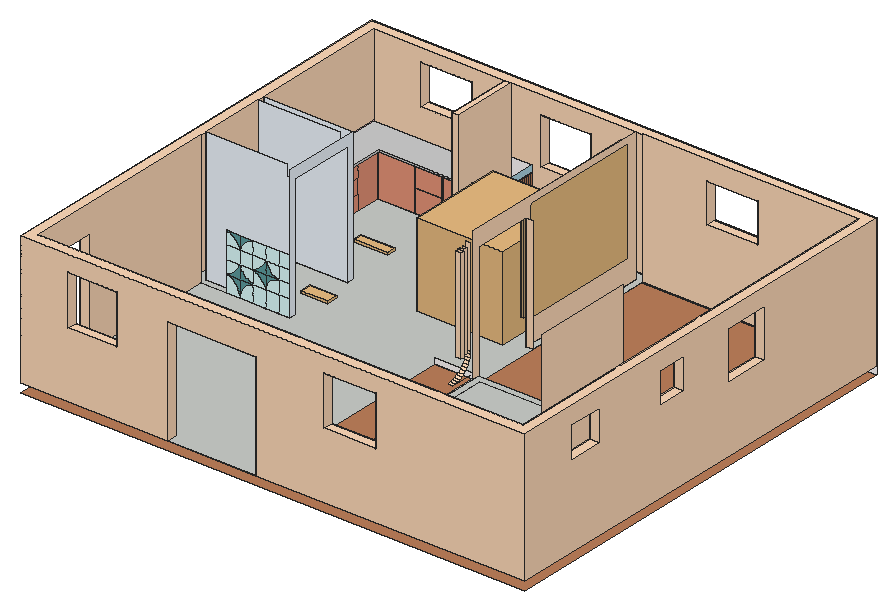
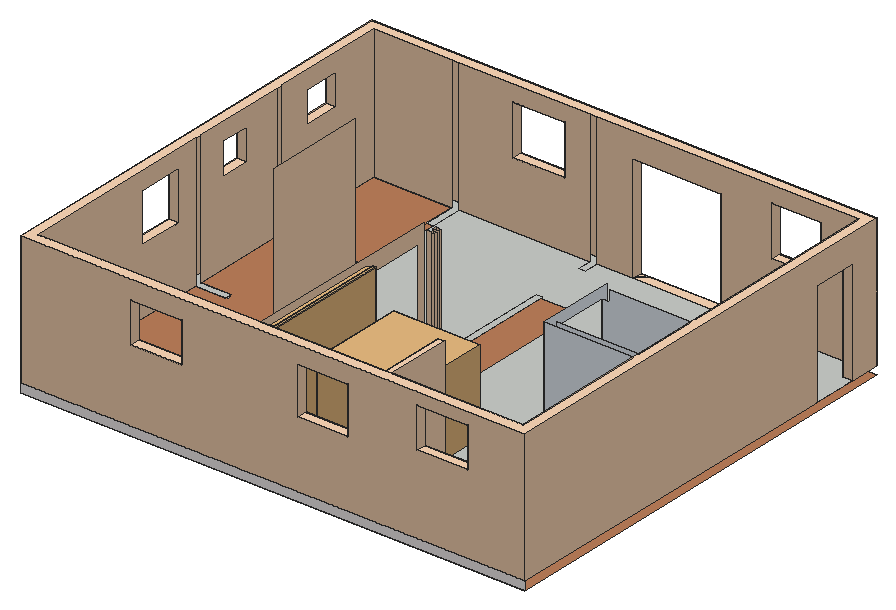
# SketchUp Ruby script. Lengths in inches.
U = 1.inch
M = Sketchup.active_model
def pt(a) = Geom::Point3d.new(a.map { |v| v * U })
def face(e, loops, mat)
  f = e.add_face(loops[0].map { |a| pt(a) })
  loops[1..].each { |l| e.add_face(l.map { |a| pt(a) }).erase! }
  f.material = f.back_material = mat if mat
  f
end
# faces: each face lists its corners as indices into pts; further lists are holes
def faces(e, pts, list, mat = nil) = list.each { |f| face(e, (f[0].is_a?(Array) ? f : [f]).map { |l| l.map { |i| pts[i] } }, mat) }
# xy, xz, yz: faces in a plane at the given z, y or x. An outline is a flat list of corners, or four numbers for a rectangle; further outlines are holes
def ring(l) = l.size == 4 ? [[l[0], l[1]], [l[2], l[1]], [l[2], l[3]], [l[0], l[3]]] : l.each_slice(2).to_a
def flat(e, list, mat, &to3) = list.each { |f| face(e, (f[0].is_a?(Array) ? f : [f]).map { |l| ring(l).map { |u, v| to3.(u, v) } }, mat) }
def xy(e, z, list, mat = nil) = flat(e, list, mat) { |x, y| [x, y, z] }
def xz(e, y, list, mat = nil) = flat(e, list, mat) { |x, z| [x, y, z] }
def yz(e, x, list, mat = nil) = flat(e, list, mat) { |y, z| [x, y, z] }
def lines(e, pts, list) = list.each { |a, b| e.add_line(pt(pts[a]), pt(pts[b])) }
# prism: a flat outline (further loops are holes) pulled along v
def prism(e, loops, v, mat = nil)
  f = face(e, loops, mat); d = Geom::Vector3d.new(v.map { |x| x * U })
  f.pushpull(f.normal.samedirection?(d) ? d.length : -d.length)
end
def box(e, o, s, mat = nil) = prism(e, [[o, [o[0] + s[0], o[1], o[2]], [o[0] + s[0], o[1] + s[1], o[2]], [o[0], o[1] + s[1], o[2]]]], [0, 0, s[2]], mat)
def at(x, y, z, deg = 0) = Geom::Transformation.translation(pt([x, y, z])) * Geom::Transformation.rotation(ORIGIN, Z_AXIS, deg.degrees)
def axes(o, x, y, z) = Geom::Transformation.new([*x, 0, *y, 0, *z, 0, *pt(o).to_a, 1])
def part(name) = M.definitions.add(name)
# library, detail: a bought-in or finely detailed component or shape, given as its bounding box
def library(name, o, s) = part(name).tap { |d| box(d.entities, o, s) }
def detail(e, o, s) = box(e.add_group.entities, o, s)
def put(e, d, t, mat = nil) = e.add_instance(d, t).tap { |i| i.material = mat if mat }
def group(e, t, mat = nil) = e.add_group.tap { |g| g.transformation = t; g.material = mat if mat }.entities
root = M.entities
M.materials.add("3D66_SU_1584934530570_001").color = [198, 166, 120]
M.materials.add("[0006_Pink]").color = [255, 192, 203]
M.materials.add("[0010_Snow]").color = [255, 250, 250]
M.materials.add("[0014_DarkSalmon]").color = [233, 150, 122]
M.materials.add("[0027_PeachPuff]").color = [255, 218, 185]
M.materials.add("[0081_CadetBlue]").color = [95, 158, 160]
M.materials.add("[0090_LightCyan]").color = [224, 255, 255]
M.materials.add("[0093_AliceBlue]").color = [240, 248, 255]
M.materials.add("[0095_LightBlue]").color = [173, 216, 230]
M.materials.add("[Basic Tile]").color = [203, 206, 202]
M.materials.add("[Carrera Marble]").color = [207, 207, 207]
M.materials.add("[Wood Veneer 02]").color = [190, 128, 91]
c1 = library("kitchen",[0.875,0,0],[30.86,8.22,2])
c2 = library("pooja",[0.875,0,0],[24.44,10.22,2])
c3 = library("Dining table and chairs",[0,0,0],[63.25,59.01,43.49])
c4 = library("Dining ar",[0.98,0,0],[40.63,10.22,2])
c5 = part("\#79\#1")
prism(c5.entities,[[[1108.05,3703.68,-100.79],[497.03,3703.68,-100.79],[497.03,5166.16,-100.79],[1108.05,5166.16,-100.79]],[[1097.77,5155.88,-100.79],[507.31,5155.88,-100.79],[507.31,3713.96,-100.79],[1097.77,3713.96,-100.79]]],[0,0,14.57],"3D66_SU_1584934530570_001")
c6 = library("\#81",[507.31,3713.96,-116.94],[590.46,1441.92,47.04])
xy(root,-7.5625,[[109.5625,138.9375,571.5625,540.9375]],"[Wood Veneer 02]")
xy(root,0,[[[109.5625,138.9375,571.5625,540.9375],[490.5625,258.9375,490.5625,347.21,492.04,347.21,492.04,350.1875,490.5625,350.1875,490.5625,351.9375,364.5625,351.9375,364.5625,531.9375,562.5625,531.9375,562.5625,351.9375,534.83,351.9375,534.83,350.1875,533.35,350.1875,533.35,348.7,535.05,348.7,535.05,345.9375,562.5625,345.9375,562.5625,258.9375],[490.5625,147.9375,490.5625,177.19,483.52,177.19,483.52,240.51,490.5625,240.51,490.5625,252.9375,562.5625,252.9375,562.5625,147.9375],[323.75,211.625,358.5625,345.9375],[118.5625,405.9375,139.41,531.9375],[244.5625,486.17,263.2,531.9375]]],"[Basic Tile]")
xy(root,6.75,[[263.2,488.05,263.89,509.17],[263.89,488.05,264.76,489.21],[263.89,490.54,264.76,491.71],[263.89,493.04,264.76,494.2],[263.89,495.53,264.76,496.7],
  [263.89,498.03,264.76,499.19],[263.89,500.52,264.76,501.6875],[263.89,503.02,264.76,504.18],[263.89,505.51,264.76,506.68],[263.89,508.01,264.76,509.17],
  [263.2,509.67,263.89,530],[263.89,510.01,264.76,511.17],[263.89,512.36,264.76,513.53],[263.89,514.71,264.76,515.88],[263.89,517.07,264.76,518.23],
  [263.89,519.42,264.76,520.59],[263.89,521.77,264.76,522.9375],[263.89,524.125,264.76,525.29],[263.89,526.48,264.76,527.65],[263.89,528.83,264.76,530]],"[0010_Snow]")
xy(root,23.08,[[354.3125,330.97,359.375,333.97],[354.3125,336.47,357.4375,339.47]],"[0027_PeachPuff]")
xy(root,44.75,[[118.58,405.9375,118.58,533.96,238.5625,533.96,238.5625,500.54,148.4,500.54,148.4,405.9375]],"[0006_Pink]")
xy(root,46.25,[[118.58,405.9375,148.4,405.9375,148.4,500.54,238.5625,500.54,238.5625,533.96,118.58,533.96]],"[Carrera Marble]")
xy(root,121.1875,[[238.5625,471.5,244.5625,531.9375]],"[0027_PeachPuff]")
xz(root,330.97,[[354.3125,23.08,359.375,110.27]],"[0027_PeachPuff]")
xz(root,333.9375,[[154.5625,0,154.5625,15.41,142.5625,15.41,144.1875,14.8125,145.74,14.05,147.22,13.14,148.59,12.09,149.85,10.9,150.98,9.59,151.97,8.17,152.82,6.66,153.5,5.07,154.03,3.42,154.38,1.72],[154.5625,0,154.6875,1.74,155,3.46,155.49,5.13,156.16,6.74,157,8.27,158,9.7,159.14,11.02,160.42,12.2,161.82,13.25,163.32,14.14,164.91,14.86,166.5625,15.41,154.5625,15.41],[142.5625,15.41,154.5625,15.41,154.5625,27.41,154.01,26.06,153.37,24.75,152.625,23.49,151.8,22.29,150.88,21.15,149.89,20.08,148.82,19.09,147.68,18.17,146.48,17.35,145.22,16.61,143.91,15.96],[154.5625,15.41,166.5625,15.41,165.19,15.93,163.86,16.55,162.59,17.27,161.37,18.09,160.22,19,159.15,19.99,158.15,21.07,157.24,22.22,156.42,23.43,155.7,24.71,155.08,26.04,154.5625,27.41],[178.5625,15.41,178.5625,27.41,166.5625,27.41,167.94,26.91,169.28,26.3,170.5625,25.58,171.79,24.77,172.94,23.86,174.02,22.87,175.02,21.79,175.93,20.63,176.74,19.41,177.45,18.125,178.0625,16.79],
  [178.5625,15.41,178.7,16.96,179.04,18.48,179.57,19.95,180.27,21.34,181.15,22.625,182.18,23.79,183.34,24.82,184.63,25.7,186.02,26.4,187.49,26.93,189.01,27.27,190.5625,27.41,178.5625,27.41],[166.5625,27.41,178.5625,27.41,178.5625,39.41,178.01,38.06,177.37,36.75,176.625,35.49,175.8,34.29,174.88,33.15,173.89,32.08,172.82,31.09,171.68,30.17,170.48,29.35,169.22,28.61,167.91,27.96],[178.5625,27.41,190.5625,27.41,189.12,27.79,187.72,28.3125,186.375,28.96,185.1,29.74,183.9,30.64,182.79,31.64,181.79,32.75,180.9,33.94,180.12,35.22,179.47,36.5625,178.95,37.96,178.5625,39.41],[154.5625,39.41,154.5625,51.41,142.5625,51.41,143.91,50.85,145.22,50.21,146.48,49.46,147.68,48.63,148.8125,47.72,149.88,46.73,150.875,45.66,151.79,44.52,152.62,43.32,153.36,42.06,154.01,40.76],[154.5625,39.41,155.0625,40.79,155.67,42.125,156.39,43.41,157.2,44.63,158.11,45.79,159.1,46.87,160.18,47.86,161.34,48.77,162.5625,49.58,163.85,50.3,165.18,50.91,166.5625,51.41,154.5625,51.41]],"[0081_CadetBlue]")
xz(root,333.9375,[[142.5625,0,154.5625,0,154.38,1.72,154.03,3.42,153.5,5.07,152.82,6.66,151.97,8.17,150.98,9.59,149.85,10.9,148.59,12.09,147.22,13.14,145.74,14.05,144.1875,14.8125,142.5625,15.41],[154.5625,0,166.5625,0,166.5625,15.41,164.91,14.86,163.32,14.14,161.82,13.25,160.42,12.2,159.14,11.02,158,9.7,157,8.27,156.16,6.74,155.49,5.13,155,3.46,154.6875,1.74],[166.5625,0,178.5625,15.41],[178.5625,0,190.5625,15.41],[190.5625,0,200.19,15.41],
  [142.5625,15.41,143.91,15.96,145.22,16.61,146.48,17.35,147.68,18.17,148.82,19.09,149.89,20.08,150.88,21.15,151.8,22.29,152.625,23.49,153.37,24.75,154.01,26.06,154.5625,27.41,142.5625,27.41],[166.5625,15.41,166.5625,27.41,154.5625,27.41,155.08,26.04,155.7,24.71,156.42,23.43,157.24,22.22,158.15,21.07,159.15,19.99,160.22,19,161.37,18.09,162.59,17.27,163.86,16.55,165.19,15.93],[166.5625,15.41,178.5625,15.41,178.0625,16.79,177.45,18.125,176.74,19.41,175.93,20.63,175.02,21.79,174.02,22.87,172.94,23.86,171.79,24.77,170.5625,25.58,169.28,26.3,167.94,26.91,166.5625,27.41],[178.5625,15.41,190.5625,15.41,190.5625,27.41,189.01,27.27,187.49,26.93,186.02,26.4,184.63,25.7,183.34,24.82,182.18,23.79,181.15,22.625,180.27,21.34,179.57,19.95,179.04,18.48,178.7,16.96],[190.5625,15.41,200.19,27.41],
  [142.5625,27.41,154.5625,39.41],[154.5625,27.41,166.5625,39.41],[166.5625,27.41,167.91,27.96,169.22,28.61,170.48,29.35,171.68,30.17,172.82,31.09,173.89,32.08,174.88,33.15,175.8,34.29,176.625,35.49,177.37,36.75,178.01,38.06,178.5625,39.41,166.5625,39.41],[190.5625,27.41,190.5625,39.41,178.5625,39.41,178.95,37.96,179.47,36.5625,180.12,35.22,180.9,33.94,181.79,32.75,182.79,31.64,183.9,30.64,185.1,29.74,186.375,28.96,187.72,28.3125,189.12,27.79],[190.5625,27.41,200.19,39.41],
  [142.5625,39.41,154.5625,39.41,154.01,40.76,153.36,42.06,152.62,43.32,151.79,44.52,150.875,45.66,149.88,46.73,148.8125,47.72,147.68,48.63,146.48,49.46,145.22,50.21,143.91,50.85,142.5625,51.41],[154.5625,39.41,166.5625,39.41,166.5625,51.41,165.18,50.91,163.85,50.3,162.5625,49.58,161.34,48.77,160.18,47.86,159.1,46.87,158.11,45.79,157.2,44.63,156.39,43.41,155.67,42.125,155.0625,40.79],[166.5625,39.41,178.5625,51.41],[178.5625,39.41,190.5625,51.41],[190.5625,39.41,200.19,51.41]],"[0090_LightCyan]")
xz(root,333.97,[[354.3125,23.08,359.375,110.27]],"[0027_PeachPuff]")
xz(root,336.47,[[354.3125,23.08,357.4375,110.27]],"[0027_PeachPuff]")
xz(root,339.47,[[354.3125,23.08,357.4375,110.27]],"[0027_PeachPuff]")
xz(root,339.9375,[[118.5625,0,118.5625,121.1875,193.07,121.1875,193.07,111.25,200.19,111.25,200.19,0]],"[0093_AliceBlue]")
xz(root,342.58,[[354.3125,24.64,358.5625,113.35]],"[0027_PeachPuff]")
xz(root,345.9375,[[323.75,0,358.5625,4.8125]],"[0010_Snow]")
xz(root,399.9375,[[118.5625,0,200.19,0,200.19,111.25,193.07,111.25,193.07,121.1875,118.5625,121.1875]],"[0093_AliceBlue]")
xz(root,405.9375,[[118.58,44.75,148.4,46.25]],"[0006_Pink]")
xz(root,405.9375,[[118.5625,0,200.19,121.1875]],"[0093_AliceBlue]")
xz(root,406.625,[[358.5625,0,364.5625,105.53]],"[0027_PeachPuff]")
xz(root,471.5,[[238.5625,0,244.5625,121.1875]],"[0027_PeachPuff]")
xz(root,486.17,[[244.5625,0,263.2,60.5]],"[0010_Snow]")
xz(root,488.05,[[263.2,6.75,263.89,54.75]],"[0010_Snow]")
xz(root,488.05,[[263.89,6.75,264.76,54.75]],"[Wood Veneer 02]")
xz(root,489.21,[[263.89,6.75,264.76,54.75]],"[Wood Veneer 02]")
xz(root,490.54,[[263.89,6.75,264.76,54.75]],"[Wood Veneer 02]")
xz(root,491.71,[[263.89,6.75,264.76,54.75]],"[Wood Veneer 02]")
xz(root,493.04,[[263.89,6.75,264.76,54.75]],"[Wood Veneer 02]")
xz(root,494.2,[[263.89,6.75,264.76,54.75]],"[Wood Veneer 02]")
xz(root,495.53,[[263.89,6.75,264.76,54.75]],"[Wood Veneer 02]")
xz(root,496.7,[[263.89,6.75,264.76,54.75]],"[Wood Veneer 02]")
xz(root,498.03,[[263.89,6.75,264.76,54.75]],"[Wood Veneer 02]")
xz(root,499.19,[[263.89,6.75,264.76,54.75]],"[Wood Veneer 02]")
xz(root,500.52,[[263.89,6.75,264.76,54.75]],"[Wood Veneer 02]")
xz(root,500.54,[[148.4,44.75,238.5625,46.25]],"[Carrera Marble]")
xz(root,501.6875,[[263.89,6.75,264.76,54.75]],"[Wood Veneer 02]")
xz(root,503.02,[[263.89,6.75,264.76,54.75]],"[Wood Veneer 02]")
xz(root,504.18,[[263.89,6.75,264.76,54.75]],"[Wood Veneer 02]")
xz(root,505.51,[[263.89,6.75,264.76,54.75]],"[Wood Veneer 02]")
xz(root,506.68,[[263.89,6.75,264.76,54.75]],"[Wood Veneer 02]")
xz(root,508.01,[[263.89,6.75,264.76,54.75]],"[Wood Veneer 02]")
xz(root,509.17,[[263.2,6.75,263.89,54.75]],"[0095_LightBlue]")
xz(root,509.17,[[263.89,6.75,264.76,54.75]],"[Wood Veneer 02]")
xz(root,509.67,[[263.2,6.75,263.89,54.75]],"[0010_Snow]")
xz(root,510.01,[[263.89,6.75,264.76,54.75]],"[Wood Veneer 02]")
xz(root,511.17,[[263.89,6.75,264.76,54.75]],"[Wood Veneer 02]")
xz(root,512.36,[[263.89,6.75,264.76,54.75]],"[Wood Veneer 02]")
xz(root,513.53,[[263.89,6.75,264.76,54.75]],"[Wood Veneer 02]")
xz(root,514.71,[[263.89,6.75,264.76,54.75]],"[Wood Veneer 02]")
xz(root,515.88,[[263.89,6.75,264.76,54.75]],"[Wood Veneer 02]")
xz(root,517.07,[[263.89,6.75,264.76,54.75]],"[Wood Veneer 02]")
xz(root,518.23,[[263.89,6.75,264.76,54.75]],"[Wood Veneer 02]")
xz(root,519.42,[[263.89,6.75,264.76,54.75]],"[Wood Veneer 02]")
xz(root,520.59,[[263.89,6.75,264.76,54.75]],"[Wood Veneer 02]")
xz(root,521.77,[[263.89,6.75,264.76,54.75]],"[Wood Veneer 02]")
xz(root,522.9375,[[263.89,6.75,264.76,54.75]],"[Wood Veneer 02]")
xz(root,524.125,[[263.89,6.75,264.76,54.75]],"[Wood Veneer 02]")
xz(root,525.29,[[263.89,6.75,264.76,54.75]],"[Wood Veneer 02]")
xz(root,526.48,[[263.89,6.75,264.76,54.75]],"[Wood Veneer 02]")
xz(root,527.65,[[263.89,6.75,264.76,54.75]],"[Wood Veneer 02]")
xz(root,528.83,[[263.89,6.75,264.76,54.75]],"[Wood Veneer 02]")
xz(root,530,[[263.2,6.75,263.89,54.75]],"[0010_Snow]")
xz(root,530,[[263.89,6.75,264.76,54.75]],"[Wood Veneer 02]")
xz(root,531.9375,[[244.5625,0,263.2,60.5]],"[0010_Snow]")
xz(root,533.96,[[118.58,44.75,238.5625,46.25]],"[0006_Pink]")
xz(root,540.9375,[[109.5625,-7.5625,571.5625,0]],"[0010_Snow]")
yz(root,118.58,[[405.9375,44.75,533.96,46.25]],"[0006_Pink]")
yz(root,148.4,[[405.9375,44.75,500.54,46.25]],"[Carrera Marble]")
yz(root,200.19,[[333.9375,0,339.9375,0,339.9375,111.25,399.9375,111.25,399.9375,0,405.9375,0,405.9375,121.1875,333.9375,121.1875]],"[0093_AliceBlue]")
yz(root,238.5625,[[500.54,44.75,533.96,46.25]],"[0006_Pink]")
yz(root,238.5625,[[471.5,0,531.9375,121.1875]],"[0027_PeachPuff]")
yz(root,244.5625,[[486.17,0,531.9375,60.5]],"[0010_Snow]")
yz(root,244.5625,[[471.5,0,531.9375,121.1875]],"[0027_PeachPuff]")
yz(root,263.2,[[[486.17,0,531.9375,60.5],[488.05,6.75,509.17,54.75],[509.67,6.75,530,54.75]]],"[0095_LightBlue]")
yz(root,263.89,[[488.05,6.75,489.21,54.75],[490.54,6.75,491.71,54.75],[493.04,6.75,494.2,54.75],[495.53,6.75,496.7,54.75],[498.03,6.75,499.19,54.75],
  [500.52,6.75,501.6875,54.75],[503.02,6.75,504.18,54.75],[505.51,6.75,506.68,54.75],[508.01,6.75,509.17,54.75],[510.01,6.75,511.17,54.75],
  [512.36,6.75,513.53,54.75],[514.71,6.75,515.88,54.75],[517.07,6.75,518.23,54.75],[519.42,6.75,520.59,54.75],[521.77,6.75,522.9375,54.75],
  [524.125,6.75,525.29,54.75]],"[0010_Snow]")
yz(root,263.89,[[489.21,6.75,490.54,54.75],[491.71,6.75,493.04,54.75],[494.2,6.75,495.53,54.75],[496.7,6.75,498.03,54.75],[499.19,6.75,500.52,54.75],
  [501.6875,6.75,503.02,54.75],[504.18,6.75,505.51,54.75],[506.68,6.75,508.01,54.75],[509.67,6.75,510.01,54.75],[511.17,6.75,512.36,54.75],
  [513.53,6.75,514.71,54.75],[515.88,6.75,517.07,54.75],[518.23,6.75,519.42,54.75],[520.59,6.75,521.77,54.75],[522.9375,6.75,524.125,54.75],
  [525.29,6.75,526.48,54.75],[526.48,6.75,527.65,54.75],[527.65,6.75,528.83,54.75],[528.83,6.75,530,54.75]],"[0095_LightBlue]")
yz(root,264.76,[[488.05,6.75,489.21,54.75],[490.54,6.75,491.71,54.75],[493.04,6.75,494.2,54.75],[495.53,6.75,496.7,54.75],[498.03,6.75,499.19,54.75],
  [500.52,6.75,501.6875,54.75],[503.02,6.75,504.18,54.75],[505.51,6.75,506.68,54.75],[508.01,6.75,509.17,54.75],[510.01,6.75,511.17,54.75],
  [512.36,6.75,513.53,54.75],[514.71,6.75,515.88,54.75],[517.07,6.75,518.23,54.75],[519.42,6.75,520.59,54.75],[521.77,6.75,522.9375,54.75],
  [524.125,6.75,525.29,54.75],[526.48,6.75,527.65,54.75],[528.83,6.75,530,54.75]],"[Wood Veneer 02]")
yz(root,357.4375,[[336.47,23.08,339.47,110.27]],"[0027_PeachPuff]")
yz(root,358.5625,[[345.9375,0,345.9375,121.1875,531.9375,121.1875,531.9375,0,406.625,0,406.625,105.53,351.9375,105.53,351.9375,0]],"[0027_PeachPuff]")
yz(root,359.375,[[330.97,23.08,333.97,110.27]],"[0027_PeachPuff]")
p = [[354.3125,322.76,4.8125],[354.3125,325.34,4.98],[358.5625,325.34,4.98],[358.5625,322.76,4.8125],[354.3125,327.89,5.49],[358.5625,327.89,5.49],
  [354.3125,330.34,6.32],[358.5625,330.34,6.32],[354.3125,332.67,7.47],[358.5625,332.67,7.47],[354.3125,334.83,8.91],[358.5625,334.83,8.91],
  [354.3125,336.78,10.62],[358.5625,336.78,10.62],[354.3125,338.49,12.57],[358.5625,338.49,12.57],[354.3125,339.93,14.73],[358.5625,339.93,14.73],
  [354.3125,341.08,17.05],[358.5625,341.08,17.05],[354.3125,341.91,19.51],[358.5625,341.91,19.51],[354.3125,342.42,22.05],[358.5625,342.42,22.05],
  [354.3125,342.58,24.64],[358.5625,342.58,24.64],[358.5625,342.58,4.8125]]
faces(root,p,[[0,1,2,3],[1,4,5,2],[4,6,7,5],[6,8,9,7],[8,10,11,9],[10,12,13,11],[12,14,15,13],[14,16,17,15],
  [16,18,19,17],[18,20,21,19],[20,22,23,21],[22,24,25,23]],"[0027_PeachPuff]")
lines(root,p,[[3,26]])
g1 = group(root,at(118.5625,405.9375,0),"[0010_Snow]")
g2 = group(g1,at(0,0,0))
xy(g2,0,[[20.85,102.47,120,126]],"[0014_DarkSalmon]")
xy(g2,4.5,[[20.85,0,20.85,102.47,29.52,102.47,29.52,97.28,26.52,97.28,26.52,0],[29.52,97.28,120,102.47],[20.85,102.47,120,126]],"[0014_DarkSalmon]")
xy(g2,5,[[26.52,1,27.65,24.73],[26.52,25.1875,27.65,38.75],[26.52,39.25,27.65,73],[26.52,73.5,27.65,95.78],[28.02,95.97,61.46,97.28],
  [61.96,95.97,86.46,97.28],[86.96,95.97,118.5,97.28]],"[0014_DarkSalmon]")
xy(g2,17.75,[[26.52,39.25,27.65,73]],"[0014_DarkSalmon]")
xy(g2,18.25,[[26.52,39.25,27.65,73]],"[0014_DarkSalmon]")
xy(g2,25.68,[[61.96,95.97,86.46,97.28]],"[0014_DarkSalmon]")
xy(g2,26.18,[[61.96,95.97,86.46,97.28]],"[0014_DarkSalmon]")
xy(g2,31.75,[[26.52,39.25,27.65,73]],"[0014_DarkSalmon]")
xy(g2,32.25,[[26.52,39.25,27.65,73]],"[0014_DarkSalmon]")
xy(g2,44.25,[[26.52,1,27.65,24.73],[26.52,25.1875,27.65,38.75],[26.52,39.25,27.65,73],[26.52,73.5,27.65,95.78],[28.02,95.97,61.46,97.28],
  [61.96,95.97,86.46,97.28],[86.96,95.97,118.5,97.28]],"[0014_DarkSalmon]")
xy(g2,44.75,[[0,0,26.52,0,26.52,97.28,120,97.28,120,126,0,126]],"[0014_DarkSalmon]")
xz(g2,0,[[0,4.5,20.85,44.75],[20.85,4.5,26.52,44.75]],"[0014_DarkSalmon]")
xz(g2,1,[[26.52,5,27.65,44.25]],"[0014_DarkSalmon]")
xz(g2,24.73,[[26.52,5,27.65,44.25]],"[0014_DarkSalmon]")
xz(g2,25.1875,[[26.52,5,27.65,44.25]],"[0014_DarkSalmon]")
xz(g2,38.75,[[26.52,5,27.65,44.25]],"[0014_DarkSalmon]")
xz(g2,39.25,[[26.52,5,27.65,17.75],[26.52,18.25,27.65,31.75],[26.52,32.25,27.65,44.25]],"[0014_DarkSalmon]")
xz(g2,73,[[26.52,5,27.65,17.75],[26.52,18.25,27.65,31.75],[26.52,32.25,27.65,44.25]],"[0014_DarkSalmon]")
xz(g2,73.5,[[26.52,5,27.65,44.25]],"[0014_DarkSalmon]")
xz(g2,95.78,[[26.52,5,27.65,44.25]],"[0014_DarkSalmon]")
xz(g2,95.97,[[28.02,5,61.46,44.25],[61.96,5,86.46,25.68],[86.96,5,118.5,44.25],[61.96,26.18,86.46,44.25]],"[0014_DarkSalmon]")
xz(g2,97.28,[[[26.52,4.5,120,44.75],[28.02,5,61.46,44.25],[86.96,5,118.5,44.25],[61.96,5,86.46,44.25]],[61.96,25.68,86.46,26.18]],"[0014_DarkSalmon]")
xz(g2,102.47,[[20.85,0,120,4.5]],"[0014_DarkSalmon]")
xz(g2,126,[[20.85,0,120,4.5],[0,4.5,120,44.75]],"[0014_DarkSalmon]")
yz(g2,0,[[0,4.5,126,44.75]],"[0014_DarkSalmon]")
yz(g2,20.85,[[0,0,102.47,4.5]],"[0014_DarkSalmon]")
yz(g2,26.52,[[0,4.5,1,44.75],[1,4.5,24.73,5],[24.73,4.5,25.1875,44.75],[25.1875,4.5,38.75,5],[[38.75,4.5,97.28,44.75],[73.5,5,95.78,44.25],[39.25,18.25,73,31.75],[39.25,5,73,17.75],[39.25,32.25,73,44.25]],
  [1,44.25,24.73,44.75],[25.1875,44.25,38.75,44.75]],"[0014_DarkSalmon]")
yz(g2,27.65,[[1,5,24.73,44.25],[25.1875,5,38.75,44.25],[39.25,5,73,17.75],[73.5,5,95.78,44.25],[39.25,18.25,73,31.75],
  [39.25,32.25,73,44.25]],"[0014_DarkSalmon]")
yz(g2,28.02,[[95.97,5,97.28,44.25]],"[0014_DarkSalmon]")
yz(g2,61.46,[[95.97,5,97.28,44.25]],"[0014_DarkSalmon]")
yz(g2,61.96,[[95.97,5,97.28,25.68],[95.97,26.18,97.28,44.25]],"[0014_DarkSalmon]")
yz(g2,86.46,[[95.97,5,97.28,25.68],[95.97,26.18,97.28,44.25]],"[0014_DarkSalmon]")
yz(g2,86.96,[[95.97,5,97.28,44.25]],"[0014_DarkSalmon]")
yz(g2,118.5,[[95.97,5,97.28,44.25]],"[0014_DarkSalmon]")
yz(g2,120,[[102.47,0,126,4.5],[97.28,4.5,126,44.75]],"[0014_DarkSalmon]")
put(root,c1,at(165.74,449.02,0))
put(root,c2,at(183.17,367.12,0))
put(root,c3,axes([265.26,397.9375,0],[1.25,0,0],[0,1.484,0],[0,0,1.7625]),"[0006_Pink]")
put(root,c4,at(289.2,501.64,0))
g3 = group(root,at(109.5625,138.9375,0),"[0027_PeachPuff]")
xy(g3,0,[[135,0,215.99,9]])
xy(g3,60.59,[[43.83,0,88.47,9],[277.57,0,325.5625,9],[453,232.22,462,274.68]])
xy(g3,61.625,[[162.09,393,208.3,402]])
xy(g3,67.48,[[313.84,393,360.72,402]])
xy(g3,72.6875,[[52.38,393,98.79,402]])
xy(g3,76.09,[[453,52.35,462,85.45],[453,154.42,462,181.83]])
xy(g3,95.4375,[[0,27,9,68.4375]])
xy(g3,97.6875,[[135,0,215.99,9]])
xy(g3,103.875,[[313.84,393,360.72,402]])
xy(g3,104.9375,[[453,52.35,462,85.45],[453,154.42,462,181.83],[453,232.22,462,274.68],[162.09,393,208.3,402]])
xy(g3,106.41,[[43.83,0,88.47,9],[277.57,0,325.5625,9]])
xy(g3,109.625,[[52.38,393,98.79,402]])
xy(g3,121.1875,[[[0,0,462,402],[9,9,453,393]]])
xz(g3,0,[[[0,0,135,0,135,97.6875,215.99,97.6875,215.99,0,462,0,462,121.1875,0,121.1875],[277.57,60.59,325.5625,106.41],[43.83,60.59,88.47,106.41]]])
xz(g3,9,[[[9,0,9,121.1875,249,121.1875,249,0,215.99,0,215.99,97.6875,135,97.6875,135,0],[43.83,60.59,88.47,106.41]],[[255,0,375,121.1875],[277.57,60.59,325.5625,106.41]],[381,0,453,121.1875]])
xz(g3,27,[[0,0,9,95.4375]])
xz(g3,52.35,[[453,76.09,462,104.9375]])
xz(g3,68.4375,[[0,0,9,95.4375]])
xz(g3,85.45,[[453,76.09,462,104.9375]])
xz(g3,154.42,[[453,76.09,462,104.9375]])
xz(g3,181.83,[[453,76.09,462,104.9375]])
xz(g3,232.22,[[453,60.59,462,104.9375]])
xz(g3,274.68,[[453,60.59,462,104.9375]])
xz(g3,393,[[[9,0,129,121.1875],[52.38,72.6875,98.79,109.625]],[[135,0,249,121.1875],[162.09,61.625,208.3,104.9375]],[[255,0,453,121.1875],[313.84,67.48,360.72,103.875]]])
xz(g3,402,[[[0,0,462,121.1875],[162.09,61.625,208.3,104.9375],[52.38,72.6875,98.79,109.625],[313.84,67.48,360.72,103.875]]])
yz(g3,0,[[0,0,0,121.1875,402,121.1875,402,0,68.4375,0,68.4375,95.4375,27,95.4375,27,0]])
yz(g3,9,[[9,0,27,0,27,95.4375,68.4375,95.4375,68.4375,0,195,0,195,121.1875,9,121.1875],[201,0,261,121.1875],[267,0,393,121.1875]])
yz(g3,43.83,[[0,60.59,9,106.41]])
yz(g3,52.38,[[393,72.6875,402,109.625]])
yz(g3,88.47,[[0,60.59,9,106.41]])
yz(g3,98.79,[[393,72.6875,402,109.625]])
yz(g3,135,[[0,0,9,97.6875]])
yz(g3,162.09,[[393,61.625,402,104.9375]])
yz(g3,208.3,[[393,61.625,402,104.9375]])
yz(g3,215.99,[[0,0,9,97.6875]])
yz(g3,277.57,[[0,60.59,9,106.41]])
yz(g3,313.84,[[393,67.48,402,103.875]])
yz(g3,325.5625,[[0,60.59,9,106.41]])
yz(g3,360.72,[[393,67.48,402,103.875]])
yz(g3,381,[[120,0,213,121.1875]])
yz(g3,453,[[[9,0,114,121.1875],[52.35,76.09,85.45,104.9375]],[[120,0,207,121.1875],[154.42,76.09,181.83,104.9375]],[[213,0,393,121.1875],[232.22,60.59,274.68,104.9375]]])
yz(g3,462,[[[0,0,402,121.1875],[232.22,60.59,274.68,104.9375],[52.35,76.09,85.45,104.9375],[154.42,76.09,181.83,104.9375]]])
p = [[0,68.4375,0],[0,27,0],[135,332.5625,0],[129,332.5625,0],[425.27,213,0],[453,213,0],
  [375,107.26,0],[375,207,0],[453,207,0],[425.27,207,0],[381,213,0],[249,213,0],
  [255,393,0],[255,267.6875,0],[381,107.26,0],[249,207,0],[249,21.68,0],[249,9,0],
  [375,21,0],[375,9,0],[249,70.55,0],[255,70.55,0],[135,393,0],[9,201,0],
  [90.63,201,0],[90.63,267,0],[9,267,0],[453,120,0],[381,120,0],[249,267.6875,0],
  [255,207,0],[381,114,0],[381,21,0],[381,9,0],[90.63,195,0],[9,195,0],
  [129,393,0],[375,68.84,0],[90.63,261,0],[249,393,0],[255,9,0],[255,21.68,0],
  [381,68.84,0],[9,261,0],[453,114,0]]
lines(g3,p,[[0,1],[2,3],[4,5],[6,7],[8,9],[10,11],[12,13],[9,4],[14,6],[15,11],[16,17],[18,19],
  [20,21],[22,2],[23,24],[25,26],[27,28],[29,13],[21,30],[31,14],[32,33],[34,35],[3,36],[30,7],
  [18,37],[38,25],[29,39],[40,41],[42,32],[41,16],[43,38],[24,34],[37,42],[15,20],[31,44]])
put(root,c5,axes([367.77,316.67,-219.49],[0,0.18694,0],[0,0,0.06481],[0.15997,0,0]),"3D66_SU_1584934530570_001")
put(root,c6,axes([369.75,316.67,-219.49],[0,0.18694,0],[0,0,0.06481],[0.16002,0,0]),"3D66_SU_1584934530570_001")
